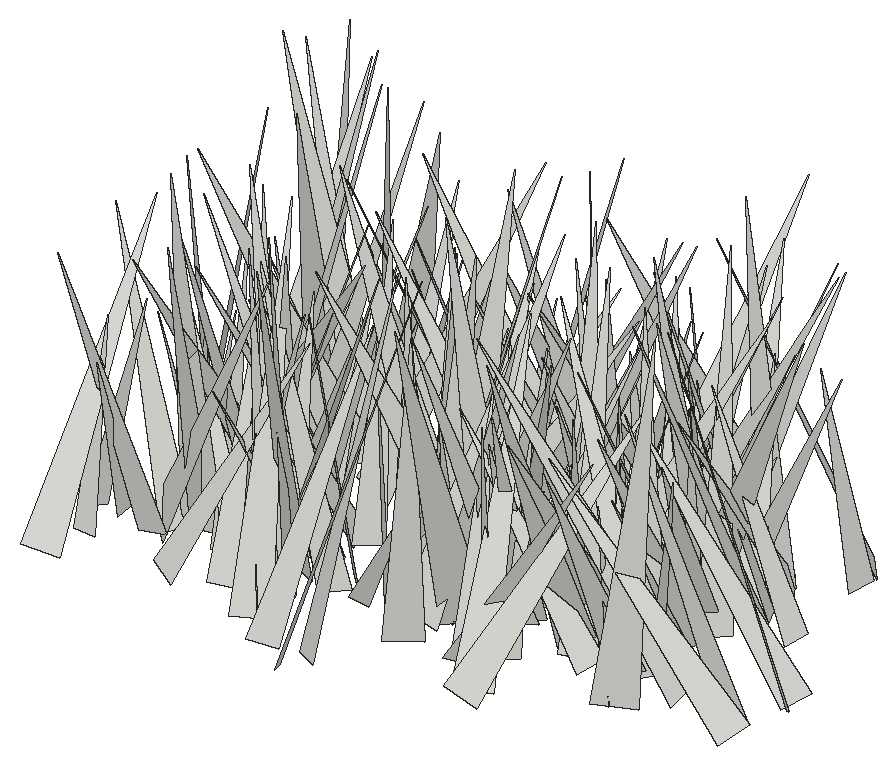
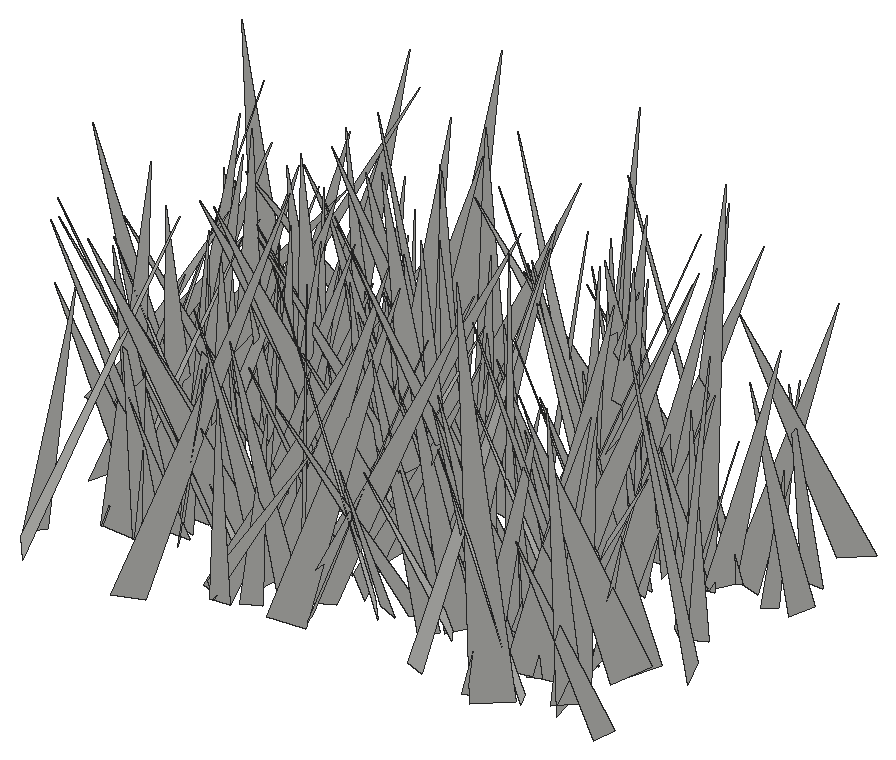
# SketchUp Ruby script. Lengths in inches.
U = 1.inch
M = Sketchup.active_model
def pt(a) = Geom::Point3d.new(a.map { |v| v * U })
def face(e, loops, mat)
  f = e.add_face(loops[0].map { |a| pt(a) })
  loops[1..].each { |l| e.add_face(l.map { |a| pt(a) }).erase! }
  f.material = f.back_material = mat if mat
  f
end
# faces: each face lists its corners as indices into pts; further lists are holes
def faces(e, pts, list, mat = nil) = list.each { |f| face(e, (f[0].is_a?(Array) ? f : [f]).map { |l| l.map { |i| pts[i] } }, mat) }
# xy, xz, yz: faces in a plane at the given z, y or x. An outline is a flat list of corners, or four numbers for a rectangle; further outlines are holes
def ring(l) = l.size == 4 ? [[l[0], l[1]], [l[2], l[1]], [l[2], l[3]], [l[0], l[3]]] : l.each_slice(2).to_a
def flat(e, list, mat, &to3) = list.each { |f| face(e, (f[0].is_a?(Array) ? f : [f]).map { |l| ring(l).map { |u, v| to3.(u, v) } }, mat) }
def xy(e, z, list, mat = nil) = flat(e, list, mat) { |x, y| [x, y, z] }
def xz(e, y, list, mat = nil) = flat(e, list, mat) { |x, z| [x, y, z] }
def yz(e, x, list, mat = nil) = flat(e, list, mat) { |y, z| [x, y, z] }
def lines(e, pts, list) = list.each { |a, b| e.add_line(pt(pts[a]), pt(pts[b])) }
# prism: a flat outline (further loops are holes) pulled along v
def prism(e, loops, v, mat = nil)
  f = face(e, loops, mat); d = Geom::Vector3d.new(v.map { |x| x * U })
  f.pushpull(f.normal.samedirection?(d) ? d.length : -d.length)
end
def box(e, o, s, mat = nil) = prism(e, [[o, [o[0] + s[0], o[1], o[2]], [o[0] + s[0], o[1] + s[1], o[2]], [o[0], o[1] + s[1], o[2]]]], [0, 0, s[2]], mat)
def at(x, y, z, deg = 0) = Geom::Transformation.translation(pt([x, y, z])) * Geom::Transformation.rotation(ORIGIN, Z_AXIS, deg.degrees)
def axes(o, x, y, z) = Geom::Transformation.new([*x, 0, *y, 0, *z, 0, *pt(o).to_a, 1])
def part(name) = M.definitions.add(name)
# library, detail: a bought-in or finely detailed component or shape, given as its bounding box
def library(name, o, s) = part(name).tap { |d| box(d.entities, o, s) }
def detail(e, o, s) = box(e.add_group.entities, o, s)
def put(e, d, t, mat = nil) = e.add_instance(d, t).tap { |i| i.material = mat if mat }
def group(e, t, mat = nil) = e.add_group.tap { |g| g.transformation = t; g.material = mat if mat }.entities
root = M.entities
c1 = part("fur_instance\#9")
p = [[0.8125,0,1.79],[0.67,-0.02,1.48],[0,-0.11,0],[0,0.11,0]]
faces(c1.entities,p,[[0,1,2,3]])
put(root,c1,axes([514.23,95.24,-21.86],[6.2923,4.31715,0.79405],[3.75537,-6.01297,2.93303],[-2.27277,2.01685,7.04472]))
put(root,c1,axes([510.16,101.49,-21.86],[-1.88375,-7.99896,1.23534],[-7.80751,2.13018,1.88761],[2.13359,0.73274,7.99805]))
put(root,c1,axes([516.61,99.59,-21.86],[4.01557,-5.25956,2.05629],[-5.53772,-4.16187,0.169],[-1.10676,1.74125,6.61508]))
put(root,c1,axes([514.66,96.4,-21.86],[3.92721,6.27569,0.86047],[6.07775,-4.01843,1.56873],[-1.78486,0.12492,7.23508]))
put(root,c1,axes([517.48,102.09,-21.86],[4.78768,-6.87101,0.53821],[-6.76798,-4.81092,-1.21319],[-1.30189,-0.25808,8.28619]))
put(root,c1,axes([504.49,100.22,-21.86],[-0.64276,-5.9949,1.38637],[-6.03632,0.34404,-1.31091],[-1.1932,1.48889,5.88502]))
put(root,c1,axes([502.57,98.64,-21.86],[0.04059,4.23783,1.33242],[4.44047,0.00019,-0.13586],[0.12965,-1.33303,4.23585]))
put(root,c1,axes([512.75,96.24,-21.86],[-4.56425,4.1816,0.8559],[3.58274,4.43445,-2.55936],[2.31998,1.37862,5.63629]))
put(root,c1,axes([502.4,96.3,-21.66],[-2.48989,6.58556,0.19317],[6.42005,2.47161,-1.51018],[1.47984,0.3578,6.87667]))
put(root,c1,axes([506.59,98.125,-21.86],[2.28513,5.39499,0.34939],[5.12885,-2.04337,-1.99232],[1.70965,-1.08097,5.50984]))
put(root,c1,axes([504.45,100.6,-21.66],[5.46808,5.3055,1.78388],[5.41419,-4.38056,-3.56761],[1.42026,-3.72732,6.73205]))
put(root,c1,axes([502.7,100.95,-21.86],[4.01864,-1.00258,0.99057],[-0.63294,-3.95809,-1.43832],[-1.25928,-1.21004,3.88405]))
put(root,c1,axes([505.75,101.54,-21.66],[6.82649,-0.20783,2.36031],[0.47416,-6.93274,-1.9818],[-2.32152,-2.02711,6.5358]))
put(root,c1,axes([511.69,99.1875,-21.86],[-6.31517,-2.67121,2.41272],[-3.08957,6.52254,-0.86542],[1.84694,1.77736,6.80204]))
put(root,c1,axes([519.14,99.66,-21.86],[4.74645,-3.63152,0.20608],[-3.44873,-4.38539,2.15263],[1.15614,1.82746,5.57521]))
put(root,c1,axes([511.54,98.15,-21.86],[-6.71,0.21588,0.88951],[-0.0468,6.49159,-1.92847],[0.91413,1.91692,6.43053]))
put(root,c1,axes([524.76,102.46,-21.66],[3.41213,-4.67618,0.33772],[-4.46229,-3.36731,-1.54031],[-1.43828,-0.64649,5.58003]))
put(root,c1,axes([508.89,98.72,-21.86],[-1.85743,4.94831,0.92273],[4.99711,1.93095,-0.29602],[0.60509,-0.75691,5.27714]))
put(root,c1,axes([522.05,103.05,-21.86],[2.00321,-7.73932,0.37509],[-7.71802,-2.02729,-0.61059],[-0.68548,0.20889,7.97102]))
put(root,c1,axes([513.53,100.86,-21.86],[1.52564,-3.34819,0.07276],[-3.07421,-1.36842,1.48995],[1.32851,0.67846,3.36423]))
put(root,c1,axes([509.4375,102.59,-21.66],[-3.6044,-3.37024,0.34721],[-3.01204,3.4196,1.92476],[1.55135,-1.19103,4.54373]))
put(root,c1,axes([519.7,100.66,-21.86],[-2.05605,-4.2865,1.82271],[-4.5186,2.31917,0.35698],[1.13077,1.47345,4.74068]))
put(root,c1,axes([521.04,97.35,-21.66],[-1.51427,6.54379,0.36236],[5.84338,1.51647,-2.96661],[2.96773,0.35306,6.02606]))
put(root,c1,axes([511.43,97.2,-21.66],[-6.67493,4.02137,0.12146],[3.83511,6.43107,-2.16198],[1.21576,1.79188,7.48679]))
put(root,c1,axes([505.81,101.47,-21.86],[1.30407,-7.61557,2.3618],[-7.95747,-1.39423,-0.10194],[-0.50366,2.30972,7.72574]))
put(root,c1,axes([525.61,100.57,-21.86],[-3.8242,6.03816,3.67075],[6.53219,4.61268,-0.78232],[2.69524,-2.61192,7.10435]))
put(root,c1,axes([501.59,100.47,-21.86],[4.23339,-1.74729,1.15695],[-1.93705,-4.25778,0.65751],[-0.79963,1.0637,4.53236]))
put(root,c1,axes([520.42,100.1,-21.86],[2.97809,2.23148,0.68885],[2.24903,-3.04112,0.12836],[-0.62921,-0.30835,3.71915]))
put(root,c1,axes([520.84,98.29,-21.86],[-3.78371,6.02543,0.57396],[5.96039,3.82698,-0.88298],[1.05307,-0.01122,7.05993]))
put(root,c1,axes([527.21,102.7,-21.66],[-8.16776,0.06376,0.0825],[0.08376,7.86119,2.21763],[0.06209,-2.2183,7.8612]))
put(root,c1,axes([530.3125,101.64,-21.86],[-5.02457,3.67244,0.21301],[3.24783,4.25941,3.17608],[-1.72736,-2.67378,5.35216]))
put(root,c1,axes([512.55,101.92,-21.86],[-3.95359,-4.39819,1.62013],[-4.4402,4.19331,0.54823],[1.50116,0.81969,5.8885]))
put(root,c1,axes([525.42,100.88,-21.86],[-3.75742,-0.36081,1.22113],[-0.40687,3.94545,-0.08619],[1.20657,0.20686,3.77372]))
put(root,c1,axes([508.95,102.55,-21.66],[8.07507,1.50255,0.4439],[1.56674,-7.73574,-2.31627],[0.00564,-2.35841,7.88031]))
put(root,c1,axes([522.47,104.77,-21.66],[4.86562,-4.5964,0.06859],[-4.19123,-4.47675,-2.68294],[-1.88818,-1.90726,6.13213]))
put(root,c1,axes([519.1,103.25,-21.86],[1.34944,-6.66989,1.0863],[-6.57389,-1.5523,-1.36482],[-1.56569,0.76902,6.66676]))
put(root,c1,axes([507.2,104.64,-21.66],[2.70234,-6.75975,0.1599],[-6.39067,-2.60962,-2.31767],[-2.20886,-0.71979,6.90111]))
put(root,c1,axes([511.02,98.98,-21.66],[-7.30125,2.0292,0.54339],[1.84392,7.1322,-1.85816],[1.00641,1.65384,7.34664]))
put(root,c1,axes([516.47,102.11,-21.66],[3.82304,5.79974,2.60132],[6.29108,-3.01834,-2.51622],[0.9089,-3.50316,6.47466]))
put(root,c1,axes([518.97,100.33,-21.86],[-2.07994,4.49979,1.08625],[4.57933,2.1742,-0.23818],[0.67657,-0.88257,4.95151]))
put(root,c1,axes([523.32,102.07,-21.66],[-5.14523,1.96025,0.06602],[1.88898,4.90265,1.64806],[-0.52792,-1.56261,5.25356]))
put(root,c1,axes([519.2,103.61,-21.86],[3.45501,-4.88886,0.26504],[-4.85303,-3.46254,-0.60598],[-0.64754,-0.13474,5.95575]))
put(root,c1,axes([505.04,100.95,-21.86],[-5.78073,2.46703,0.60773],[2.49572,5.79658,0.20851],[0.47643,-0.43109,6.28168]))
put(root,c1,axes([512.35,100.93,-21.86],[-1.88222,6.06948,1.49765],[6.0067,1.32242,2.18977],[-1.73238,-2.00921,5.96542]))
put(root,c1,axes([507.48,102.99,-21.86],[-1.29627,-6.42722,1.30707],[-6.54569,1.18361,-0.67151],[-0.41416,1.4099,6.52216]))
put(root,c1,axes([507.01,102.66,-21.86],[3.94876,4.2171,2.00571],[4.64379,-3.26946,-2.26834],[0.4919,-2.98768,5.31331]))
put(root,c1,axes([510.23,104.85,-21.86],[-6.16351,-3.9605,0.27898],[-3.73191,5.95492,2.08903],[1.35509,-1.6142,7.02213]))
put(root,c1,axes([514.91,100.79,-21.66],[-3.90269,-1.36809,1.23152],[-1.73858,3.68797,-1.41263],[0.60468,1.77384,3.88679]))
put(root,c1,axes([519,103.51,-21.86],[3.0521,-3.8403,0.46149],[-3.78154,-3.08617,-0.67208],[-0.8129,-0.06212,4.85917]))
put(root,c1,axes([507.91,100.9,-21.86],[-2.49681,4.68547,0.3153],[4.52882,2.308,1.56527],[-1.24213,-1.0033,5.07323]))
put(root,c1,axes([529.72,102.38,-21.86],[-0.80032,5.57612,2.90873],[5.9333,-0.30294,2.21326],[-2.08561,-3.00158,5.18026]))
put(root,c1,axes([509.59,101.84,-21.86],[3.71191,-5.65782,4.04126],[-6.28277,-4.69165,-0.79764],[-2.97818,2.84578,6.7196]))
put(root,c1,axes([520.45,100.97,-21.86],[-3.95695,1.67084,0.9926],[1.45221,4.03835,-1.00857],[1.29152,0.5783,4.17516]))
put(root,c1,axes([516.375,104.63,-21.66],[-6.66712,2.68909,2.42043],[3.53397,5.92752,3.14894],[0.77508,-3.89533,6.46266]))
put(root,c1,axes([511.07,102.29,-21.86],[-7.40149,0.22253,0.007],[0.22253,7.40149,0.00759],[0.00677,-0.0078,7.40483]))
put(root,c1,axes([507.7,103.78,-21.86],[5.14782,-4.26055,1.16689],[-4.27581,-5.25589,-0.32723],[-1.10966,0.4872,6.67423]))
put(root,c1,axes([518.1,104.32,-21.86],[7.05622,-1.23215,0.51957],[-1.10047,-6.93599,-1.50315],[-0.75967,-1.39725,7.0035]))
put(root,c1,axes([505.01,102.8,-21.86],[-3.79015,-1.11399,0.60809],[-1.15598,3.82064,-0.20588],[0.52388,0.37109,3.9451]))
put(root,c1,axes([526.59,104.18,-21.66],[-3.56897,-0.50146,0.42511],[-0.28446,3.29362,1.49696],[0.59267,-1.43888,3.27843]))
put(root,c1,axes([524.74,104.09,-21.86],[-1.98967,-4.65459,1.69235],[-4.24096,2.54317,2.00863],[2.55803,0.59592,4.64644]))
put(root,c1,axes([515.72,103.68,-21.86],[0.0585,-4.06465,0.78718],[-4.11626,0.02739,0.44734],[0.44434,0.78888,4.04038]))
put(root,c1,axes([520.91,104.52,-21.86],[-0.89521,-5.51634,1.09126],[-5.41102,1.14576,1.35291],[1.53027,0.82431,5.42227]))
put(root,c1,axes([505.24,101.73,-21.86],[-3.70619,1.07071,1.22273],[0.63141,3.75399,-1.37341],[1.4976,1.06701,3.605]))
put(root,c1,axes([516.2,100.95,-21.66],[0.38295,8.08113,1.09098],[7.9956,-0.1576,-1.6392],[1.60161,-1.14545,7.92239]))
put(root,c1,axes([517.57,104.03,-21.86],[3.59874,-6.83955,3.08177],[-7.12327,-4.18751,-0.97538],[-2.35281,2.21652,7.66674]))
put(root,c1,axes([515.69,103.27,-21.86],[-2.45983,6.23998,3.07468],[6.83629,2.77173,-0.15592],[1.28687,-2.79677,6.7055]))
put(root,c1,axes([503.23,104.5,-21.86],[0.91273,-4.1627,0.50654],[-4.12867,-0.80133,0.85424],[0.734,0.66898,4.1751]))
put(root,c1,axes([507.3,100.75,-21.86],[-5.60466,1.1961,0.32776],[0.92969,5.05609,-2.5538],[0.82084,2.4404,5.13039]))
put(root,c1,axes([514.85,103.875,-21.86],[7.01983,-0.71592,2.31882],[-0.6287,-7.39114,-0.37866],[-2.34397,-0.1616,7.04608]))
put(root,c1,axes([525.14,106.04,-21.86],[2.61621,-5.42084,0.25429],[-5.22177,-2.59146,-1.52055],[-1.47757,-0.43991,5.82391]))
put(root,c1,axes([526.8,104.07,-21.86],[-1.27388,-3.61865,0.59779],[-3.46584,0.98064,-1.44951],[-1.19998,1.0092,3.55195]))
put(root,c1,axes([515.02,101.59,-21.86],[-0.78819,5.89997,0.04998],[5.7265,0.75282,1.4401],[-1.42105,-0.23877,5.77555]))
put(root,c1,axes([508.61,102.98,-21.86],[-1.7521,4.37342,1.24469],[4.49457,1.86786,-0.23622],[0.6891,-1.06311,4.7054]))
put(root,c1,axes([525.22,103.1,-21.86],[-6.12251,3.37612,2.03098],[3.42132,6.417,-0.35327],[1.95387,-0.65732,6.98272]))
put(root,c1,axes([513.63,104.03,-21.86],[-0.9402,5.50023,2.63792],[6.09336,0.97222,0.14463],[0.28664,-2.62629,5.57814]))
put(root,c1,axes([512.95,103.96,-21.86],[4.20762,-3.32651,0.12048],[-3.15177,-3.91891,1.86887],[1.07075,1.53645,5.02763]))
put(root,c1,axes([519.12,101.92,-21.86],[2.4518,5.85296,0.01413],[5.81055,-2.43218,-0.76857],[0.70347,-0.30989,6.29903]))
put(root,c1,axes([521.99,104.73,-21.86],[-0.88602,-4.48963,1.06047],[-4.46813,0.56653,-1.33464],[-1.14769,1.26043,4.37728]))
put(root,c1,axes([508.05,103.17,-21.86],[4.17653,-0.25853,0.87813],[-0.4857,-4.1025,1.10224],[-0.77592,1.17643,4.03674]))
put(root,c1,axes([525.11,103.13,-21.66],[-3.78872,6.01371,0.63065],[5.87535,3.48538,2.06137],[-1.42923,-1.61377,6.8022]))
put(root,c1,axes([524.75,102.72,-21.86],[-5.22043,-0.84385,1.05571],[-1.17009,4.93002,-1.84535],[0.67639,2.01552,4.95577]))
put(root,c1,axes([530.73,104.71,-21.66],[-3.83855,4.56526,0.77541],[4.17711,2.97899,3.13921],[-1.99865,-2.54191,5.07163]))
put(root,c1,axes([522.3,102.56,-21.86],[-1.2461,7.24945,1.28302],[7.36015,1.19663,0.38699],[-0.1701,-1.32928,7.34558]))
put(root,c1,axes([518.875,103.1,-21.86],[-3.66348,3.88372,0.60062],[3.90017,3.69385,-0.09601],[0.48235,-0.37054,5.33808]))
put(root,c1,axes([522.56,104.56,-21.86],[4.15283,1.56186,1.94961],[1.7605,-4.5132,-0.13443],[-1.7723,-0.82343,4.43479]))
put(root,c1,axes([524.82,107,-21.86],[4.609,-3.3139,0.05026],[-3.15306,-4.41083,-1.68231],[-1.0211,-1.33793,5.42168]))
put(root,c1,axes([523.34,103.49,-21.86],[-1.57636,3.66287,0.67143],[3.67727,1.64614,-0.34684],[0.58749,-0.47537,3.97256]))
put(root,c1,axes([515.52,104.93,-21.86],[4.4628,-4.8312,0.78242],[-4.8199,-4.15484,1.83716],[0.84924,1.80724,6.31521]))
put(root,c1,axes([516.85,104.95,-21.86],[3.82808,-2.96393,0.87418],[-3.08142,-3.76593,0.72521],[-0.23226,1.11183,4.78677]))
put(root,c1,axes([519.26,105.05,-21.86],[3.70956,-2.15387,1.10856],[-2.28011,-3.78925,0.26761],[-0.81802,0.79458,4.28116]))
put(root,c1,axes([513.9,104.74,-21.86],[-3.05036,2.77962,1.08054],[2.93347,3.07501,0.37088],[0.53722,-1.00823,4.11016]))
put(root,c1,axes([503.76,104.83,-21.86],[-3.6941,-4.73944,2.34113],[-5.23892,3.66336,-0.85037],[0.70493,2.38895,5.94858]))
put(root,c1,axes([526.98,107.72,-21.66],[-6.21102,-4.85766,0.88936],[-4.64444,6.23147,1.60082],[1.67841,-0.73247,7.72082]))
put(root,c1,axes([524.04,107.38,-21.86],[-3.10911,-5.59083,0.18925],[-5.58666,3.11434,0.22319],[0.28707,0.05678,6.39328]))
put(root,c1,axes([518,106.27,-21.86],[-7.5943,2.08618,0.38061],[2.11361,7.33132,1.9887],[-0.17228,-2.01745,7.62041]))
put(root,c1,axes([506.6,106.07,-21.86],[-3.02688,-2.08558,0.64094],[-2.07151,3.09116,0.27563],[0.68504,0.13224,3.66547]))
put(root,c1,axes([530.96,103.97,-21.66],[-6.11447,-3.98639,0.59028],[-3.68819,5.10346,-3.73879],[-1.62389,3.41906,6.26894]))
put(root,c1,axes([503.3125,107.5625,-21.86],[2.01455,-7.63294,0.11302],[-6.59973,-1.68273,3.99311],[3.83642,1.11337,6.80994]))
put(root,c1,axes([505.19,106.36,-21.66],[6.89965,2.05968,0.48381],[2.11498,-6.67017,-1.76557],[0.05673,-1.82978,6.98071]))
put(root,c1,axes([512.9,106.66,-21.86],[-6.83352,3.26319,2.339],[3.80782,6.73136,1.73366],[1.27275,-2.61852,7.37155]))
put(root,c1,axes([520.67,104.6,-21.86],[-5.59489,5.13542,2.2708],[5.22691,5.9344,-0.54239],[2.05147,-1.11455,7.57503]))
put(root,c1,axes([508.6875,104.27,-21.86],[5.33264,0.16428,1.51785],[-0.27785,-5.31816,1.55174],[-1.50122,1.56784,5.10452]))
put(root,c1,axes([511.2,104.34,-21.86],[-5.25856,3.05312,1.43062],[2.8843,5.44607,-1.02073],[1.74617,0.1987,5.99435]))
put(root,c1,axes([515.25,102.55,-21.66],[6.25178,5.32919,0.93445],[4.93149,-6.20008,2.36594],[-2.22574,1.23164,7.86685]))
put(root,c1,axes([517.03,105.98,-21.86],[3.66382,-3.28739,1.57998],[-3.52995,-3.75957,0.36325],[-0.918,1.33625,4.90903]))
put(root,c1,axes([519.24,108.08,-21.86],[4.74802,-2.11154,0.82126],[-1.70244,-4.58339,-1.94189],[-1.49491,-1.48682,4.81989]))
put(root,c1,axes([514.86,104.5625,-21.86],[1.506,6.6666,0.93752],[6.04421,-0.91584,-3.19677],[2.9648,-1.51928,6.04088]))
put(root,c1,axes([517.52,105.71,-21.86],[-5.46904,-3.01802,0.13387],[-2.92547,5.22183,-1.79189],[-0.75368,1.63119,5.98398]))
put(root,c1,axes([513.15,106.49,-21.86],[0.6303,-6.24139,2.24897],[-6.57772,-0.29373,1.02832],[0.86396,2.31708,6.18828]))
put(root,c1,axes([507.08,108.79,-21.66],[-7.12654,1.94071,2.81889],[3.04033,6.57978,3.15641],[1.57127,-3.9294,6.67765]))
put(root,c1,axes([522.04,104.65,-21.66],[-6.81045,0.95525,0.6863],[0.79996,6.71798,-1.4123],[0.86231,1.31226,6.73054]))
put(root,c1,axes([514.45,105.55,-21.86],[-3.47776,6.78239,3.15196],[7.08859,4.09761,-0.99596],[2.38486,-2.28893,7.55669]))
put(root,c1,axes([520.95,108.27,-21.86],[3.32641,-4.64571,1.36805],[-4.19977,-3.59363,-1.99171],[-2.41165,-0.14974,5.35544]))
put(root,c1,axes([523.93,108.67,-21.66],[5.76412,-4.56343,1.38579],[-4.26746,-5.90574,-1.69745],[-2.12934,-0.51736,7.15322]))
put(root,c1,axes([508.4375,105.43,-21.86],[-0.0874,4.08723,0.80677],[4.1529,0.14964,-0.30818],[0.33125,-0.79758,4.07653]))
put(root,c1,axes([507.72,106.89,-21.86],[-2.7303,-2.91554,0.15676],[-2.8364,2.59761,-1.08937],[-0.69267,0.85529,3.84294]))
put(root,c1,axes([523.67,107.51,-21.86],[0.51611,-4.80053,1.29544],[-4.96034,-0.40702,0.46794],[0.34389,1.33374,4.80546]))
put(root,c1,axes([515.18,104.63,-21.86],[-3.56356,5.20391,0.71647],[5.00613,3.62664,-1.4419],[1.59144,0.24443,6.14008]))
put(root,c1,axes([517.95,104.32,-21.86],[7.47799,-1.52657,1.95795],[-2.25093,-6.79047,3.30259],[-1.04752,3.69369,6.88067]))
put(root,c1,axes([501.84,106.5,-21.86],[6.18065,2.99725,1.89028],[2.99834,-6.44896,0.42186],[-1.88855,-0.42956,6.85609]))
put(root,c1,axes([517.27,108.51,-21.86],[4.19489,0.81761,0.41517],[0.91291,-3.90671,-1.53042],[-0.08632,-1.58339,3.99042]))
put(root,c1,axes([525.36,111.33,-21.86],[-4.76497,-3.93422,0.44703],[-3.2824,4.31602,2.99679],[2.21445,-2.06803,5.40391]))
put(root,c1,axes([523.18,108.74,-21.66],[5.01421,-5.55154,0.43768],[-5.45899,-4.78379,1.86233],[1.10028,1.565,7.24525]))
put(root,c1,axes([519.41,108.41,-21.86],[5.69628,-2.00129,2.37758],[-1.98509,-6.1627,-0.4314],[-2.39112,0.34864,6.02217]))
put(root,c1,axes([523.3,108.86,-21.86],[0.92373,-7.0899,2.33425],[-7.39568,-1.18748,-0.68009],[-1.00963,2.21177,7.11741]))
put(root,c1,axes([520.3,106.24,-21.66],[1.42855,6.69806,0.59183],[6.31436,-1.12829,-2.47201],[2.31152,-1.05735,6.38701]))
put(root,c1,axes([522.76,109.71,-21.86],[-2.364,-4.99525,1.36106],[-4.8414,2.66304,1.36474],[1.83462,0.59091,5.35523]))
put(root,c1,axes([515.41,106.84,-21.66],[7.23014,-2.66142,0.8801],[-2.79977,-6.73645,2.62947],[0.1379,2.76941,7.24182]))
put(root,c1,axes([527.68,108.53,-21.86],[-5.10669,0.68056,0.36828],[0.71376,5.09217,0.48729],[0.29888,-0.53268,5.12875]))
put(root,c1,axes([511.23,107.62,-21.86],[4.30125,1.72732,0.68489],[1.69718,-4.35514,0.32517],[-0.75649,0.05042,4.6237]))
put(root,c1,axes([522.99,107.06,-21.86],[-4.49131,4.50007,0.95246],[4.50728,4.57122,-0.34355],[0.91773,-0.42777,6.34858]))
put(root,c1,axes([505.3125,105.875,-21.86],[5.00071,5.94343,0.88428],[5.7504,-5.06729,1.53914],[-1.74336,0.3341,7.61331]))
put(root,c1,axes([525.42,106.57,-21.66],[-6.65914,2.85732,1.17721],[2.6023,6.69305,-1.52492],[1.66678,0.96593,7.084]))
put(root,c1,axes([515.25,109.05,-21.86],[-3.40667,-4.88664,0.79026],[-4.79108,3.01371,-2.01797],[-1.2447,1.77411,5.60468]))
put(root,c1,axes([509.06,107.2,-21.66],[1.74287,7.71217,1.36191],[7.45298,-1.20484,-2.71503],[2.4053,-1.85492,7.42588]))
put(root,c1,axes([508.53,108.63,-21.86],[7.01213,2.59998,3.36264],[2.81322,-7.70163,0.08845],[-3.18638,-1.07803,7.47811]))
put(root,c1,axes([509.95,112.48,-21.86],[-4.53794,-6.8341,0.16977],[-6.57814,4.42074,2.12406],[1.86058,-1.03861,7.92377]))
put(root,c1,axes([521.16,108.27,-21.86],[-3.597,-0.64897,1.74683],[-0.97146,3.89365,-0.55385],[1.59023,0.91068,3.61287]))
put(root,c1,axes([503.64,111.29,-21.66],[7.57168,-2.77915,1.4038],[-2.39268,-7.55557,-2.05259],[-1.99233,-1.48808,7.80006]))
put(root,c1,axes([510.42,109.23,-21.86],[4.08731,-3.32744,0.79787],[-3.41978,-4.01464,0.77613],[-0.11643,1.10699,5.21302]))
put(root,c1,axes([506.42,107.57,-21.86],[4.71146,3.59222,0.48874],[3.58656,-4.73541,0.23065],[-0.52868,-0.11206,5.92019]))
put(root,c1,axes([526.09,109.07,-21.66],[-5.87124,-3.56524,0.53214],[-3.58838,5.68376,-1.51131],[-0.34307,1.5651,6.70063]))
put(root,c1,axes([520.78,107.48,-21.66],[-1.18961,5.30841,0.21099],[4.92708,1.02155,2.07828],[-1.98686,-0.64508,5.02744]))
put(root,c1,axes([511.83,108.64,-21.86],[-0.91828,3.53646,1.4047],[3.57282,1.29857,-0.93362],[1.30946,-1.06309,3.53244]))
put(root,c1,axes([504.85,108.32,-21.86],[-3.94683,-0.00707,0.27926],[-0.08275,3.80753,-1.07302],[0.26682,1.07619,3.79817]))
put(root,c1,axes([516.29,108.47,-21.86],[2.1149,3.97719,0.39309],[3.90996,-1.96694,-1.13523],[0.82754,-0.87089,4.35914]))
put(root,c1,axes([506.07,109.69,-21.86],[-0.24742,-3.68689,1.2628],[-3.55064,-0.30834,-1.59591],[-1.60648,1.24932,3.33279]))
put(root,c1,axes([510.92,110.45,-21.66],[-0.06945,-5.66946,1.63507],[-5.27402,0.7929,2.5253],[2.64594,1.43164,5.07647]))
put(root,c1,axes([505.49,107.89,-21.86],[3.5873,6.66463,1.07182],[6.75002,-3.55215,-0.50434],[-0.05834,-1.18311,7.55193]))
put(root,c1,axes([505.89,110.59,-21.66],[-0.58442,-4.16845,1.10453],[-3.96593,0.95723,1.51414],[1.69333,0.80327,3.92746]))
put(root,c1,axes([515.2,111.94,-21.86],[-4.86193,-2.9811,0.43497],[-2.74592,4.72474,1.68858],[1.2394,-1.22654,5.44739]))
put(root,c1,axes([517.53,110.52,-21.66],[-1.28539,6.13898,3.44989],[6.89976,0.39684,1.86462],[-1.40785,-3.66012,5.98853]))
put(root,c1,axes([518.62,109.45,-21.86],[4.75078,2.28793,0.55209],[2.32197,-4.75936,-0.25743],[-0.38451,-0.47246,5.26671]))
put(root,c1,axes([508.31,109.76,-21.86],[4.91416,0.05831,0.74386],[0.02898,-4.96646,0.19783],[-0.74558,0.19125,4.91052]))
put(root,c1,axes([515.48,111.21,-21.66],[-6.93796,2.79801,1.11968],[3.01121,6.55067,2.28891],[0.12298,-2.54512,7.12215]))
put(root,c1,axes([506.13,110.59,-21.66],[-4.3642,6.37446,3.0679],[7.06974,4.05938,1.62241],[0.25406,-3.46117,7.553]))
put(root,c1,axes([515.68,112.75,-21.86],[3.27903,-5.74844,0.73311],[-5.41958,-3.34021,-1.9507],[-2.05188,-0.36394,6.32387]))
put(root,c1,axes([522.7,107.66,-21.86],[5.97415,4.42308,0.10738],[4.35531,-5.91092,1.16532],[-0.77872,0.87356,7.3414]))
put(root,c1,axes([523.39,106.77,-21.66],[-6.0414,2.82747,0.77084],[2.14541,5.47009,-3.25002],[1.99649,2.67784,5.82499]))
put(root,c1,axes([504.6,106.95,-21.86],[3.79972,6.90357,0.39781],[6.61789,-3.76205,2.07507],[-2.00527,0.66563,7.60206]))
put(root,c1,axes([518.92,112.7,-21.86],[0.00181,-5.98408,0.19016],[-5.68264,-0.06159,-1.88392],[-1.88493,0.17992,5.67979]))
put(root,c1,axes([508.44,109.25,-21.86],[-0.03084,5.75903,1.17934],[5.85206,0.14189,-0.53988],[0.55736,-1.17118,5.73375]))
put(root,c1,axes([519.3,110.5,-21.86],[5.75926,3.61485,0.22209],[3.58079,-5.62103,-1.36658],[0.54262,-1.27375,6.66098]))
put(root,c1,axes([506.66,112.95,-21.66],[4.42124,-3.27,0.9733],[-2.9097,-4.44582,-1.71927],[-1.78153,-0.85401,5.22344]))
put(root,c1,axes([523.77,110.25,-21.66],[4.38543,-2.43855,0.87514],[-2.59033,-4.09309,1.5752],[0.05089,1.80126,4.76417]))
put(root,c1,axes([517.07,110.04,-21.86],[-5.7993,-3.05465,2.69516],[-3.68736,5.92923,-1.21419],[1.7315,2.39584,6.44116]))
put(root,c1,axes([507.56,108.77,-21.66],[-0.98442,7.82804,0.7856],[7.24103,0.59195,3.17514],[-3.07617,-1.11168,7.22258]))
put(root,c1,axes([512.25,109.37,-21.86],[1.05381,5.0713,0.10966],[4.76326,-0.95083,-1.80217],[1.74396,-0.4674,4.856]))
put(root,c1,axes([520.4375,110.26,-21.66],[4.59981,5.90875,0.46757],[5.722,-4.27232,-2.30133],[1.54616,-1.76752,7.12569]))
put(root,c1,axes([503.27,108.29,-21.66],[-5.30404,4.85737,1.41696],[4.30663,5.41145,-2.42976],[2.65607,0.92563,6.76928]))
put(root,c1,axes([510.57,109.52,-21.86],[3.43862,2.40363,0.16823],[2.31203,-3.37399,0.94893],[-0.67841,0.6845,4.08669]))
put(root,c1,axes([513.81,109.87,-21.86],[5.53821,4.98185,1.27941],[5.04776,-5.62536,0.05401],[-0.98782,-0.81487,7.449]))
put(root,c1,axes([517.95,110.82,-21.86],[4.66394,-1.20705,1.00362],[-1.36601,-4.67089,0.73033],[-0.77347,0.97077,4.76192]))
put(root,c1,axes([524.49,111.32,-21.86],[0.36283,-7.33481,3.26148],[-7.98321,-0.67122,-0.62142],[-0.83968,3.21222,7.31744]))
put(root,c1,axes([505.93,112.98,-21.66],[3.30529,-7.09092,0.75642],[-7.06387,-3.14139,1.41833],[0.97724,1.27626,7.69379]))
put(root,c1,axes([524.51,109.45,-21.86],[-2.78795,6.31949,0.96814],[6.36227,2.84625,-0.25738],[0.62828,-0.78026,6.90234]))
put(root,c1,axes([513.32,109.84,-21.86],[1.03899,3.82207,0.22987],[3.79032,-1.06041,0.49963],[-0.54276,-0.08876,3.92914]))
put(root,c1,axes([523.58,110.94,-21.86],[2.89571,-2.97183,2.13904],[-3.49598,-3.05481,0.48854],[-1.08874,1.90494,4.12046]))
put(root,c1,axes([522.78,109.99,-21.86],[-5.03149,-1.83162,1.20846],[-2.18082,4.50919,-2.24552],[0.24343,2.5384,4.86091]))
put(root,c1,axes([521.33,114.85,-21.86],[-7.73279,0.49202,2.83462],[1.75633,7.24586,3.53356],[2.27869,-3.91518,6.89581]))
put(root,c1,axes([522.53,110.43,-21.66],[2.40606,6.39383,1.08481],[6.38564,-2.13376,-1.58675],[1.13207,-1.55339,6.64473]))
put(root,c1,axes([517.5,112.5,-21.86],[2.03457,-2.99845,1.01926],[-3.06758,-2.16697,-0.25148],[-0.78708,0.69471,3.61482]))
put(root,c1,axes([505.45,111.85,-21.86],[4.3525,2.53578,0.43229],[2.57081,-4.2585,-0.90411],[0.08934,-0.99816,4.9555]))
put(root,c1,axes([516.84,111.08,-21.86],[0.44242,5.64748,1.29703],[5.78226,-0.34572,-0.46699],[0.37666,-1.32609,5.6455]))
put(root,c1,axes([527.06,113.08,-21.86],[4.20178,-1.75309,2.00996],[-1.5081,-4.65512,-0.90755],[-2.19975,-0.15714,4.46146]))
put(root,c1,axes([519.09,112.875,-21.66],[-2.36065,-3.34559,0.0438],[-3.13879,2.19578,-1.44709],[-1.15883,0.86782,3.83035]))
put(root,c1,axes([501.26,112.34,-21.66],[2.74116,-2.85153,0.16279],[-2.64199,-2.44575,1.64616],[1.08517,1.2485,3.59657]))
put(root,c1,axes([519.53,109.78,-21.86],[-1.94232,7.80928,1.11049],[7.41359,2.19794,-2.48968],[2.69386,-0.41817,7.65238]))
put(root,c1,axes([526.61,114.43,-21.86],[-5.605,-5.08718,0.25266],[-5.09303,5.60246,-0.18084],[0.06544,0.30374,7.56721]))
put(root,c1,axes([503.97,110.97,-21.86],[-7.13651,-0.0123,2.39844],[-0.61978,7.28244,-1.80677],[2.31701,1.91008,6.90402]))
put(root,c1,axes([518.53,113.05,-21.86],[0.16475,-3.83195,1.51207],[-4.1166,-0.0965,0.20397],[0.15418,1.51796,3.83006]))
